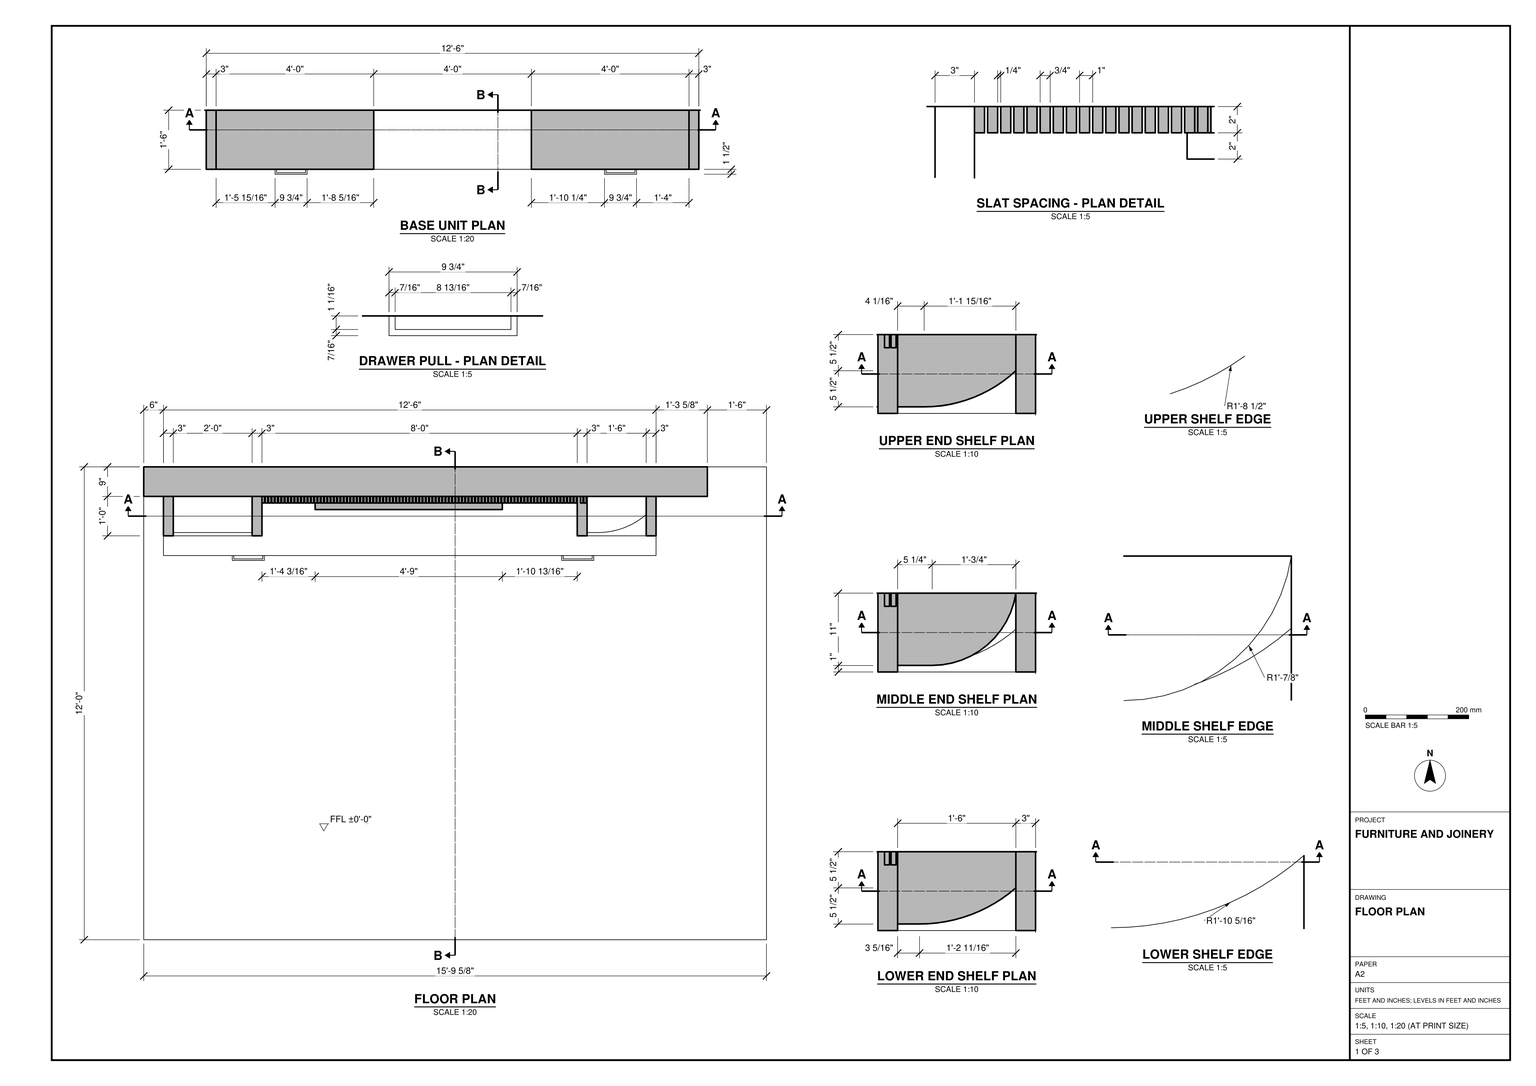
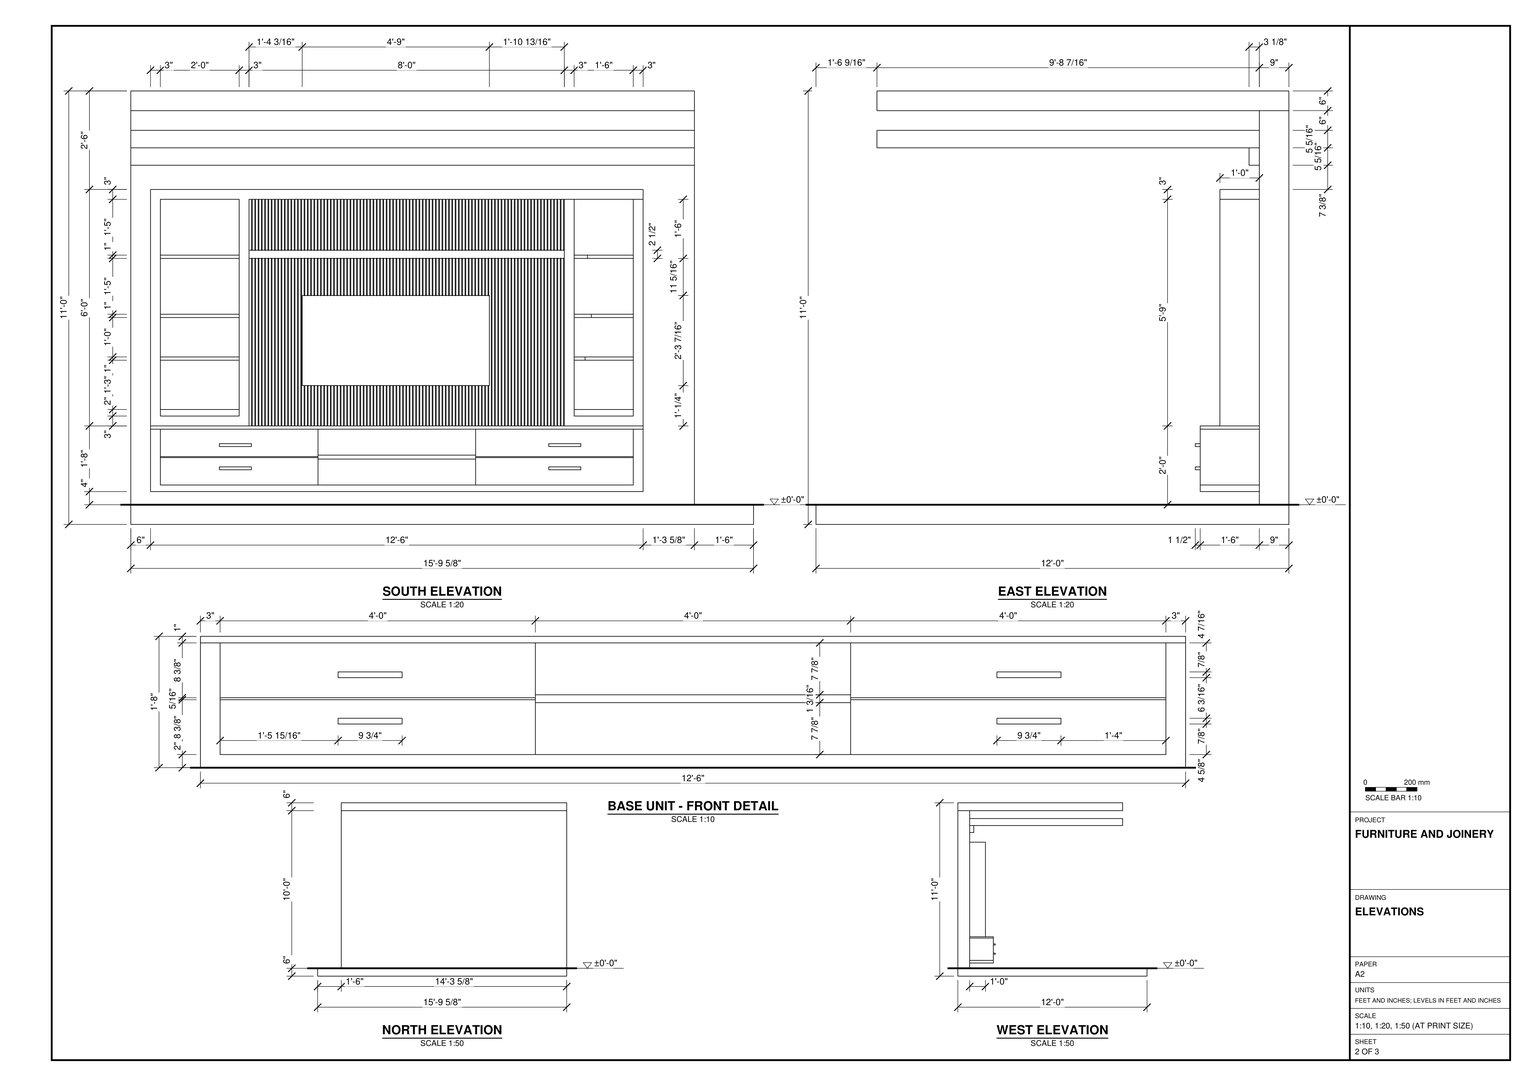
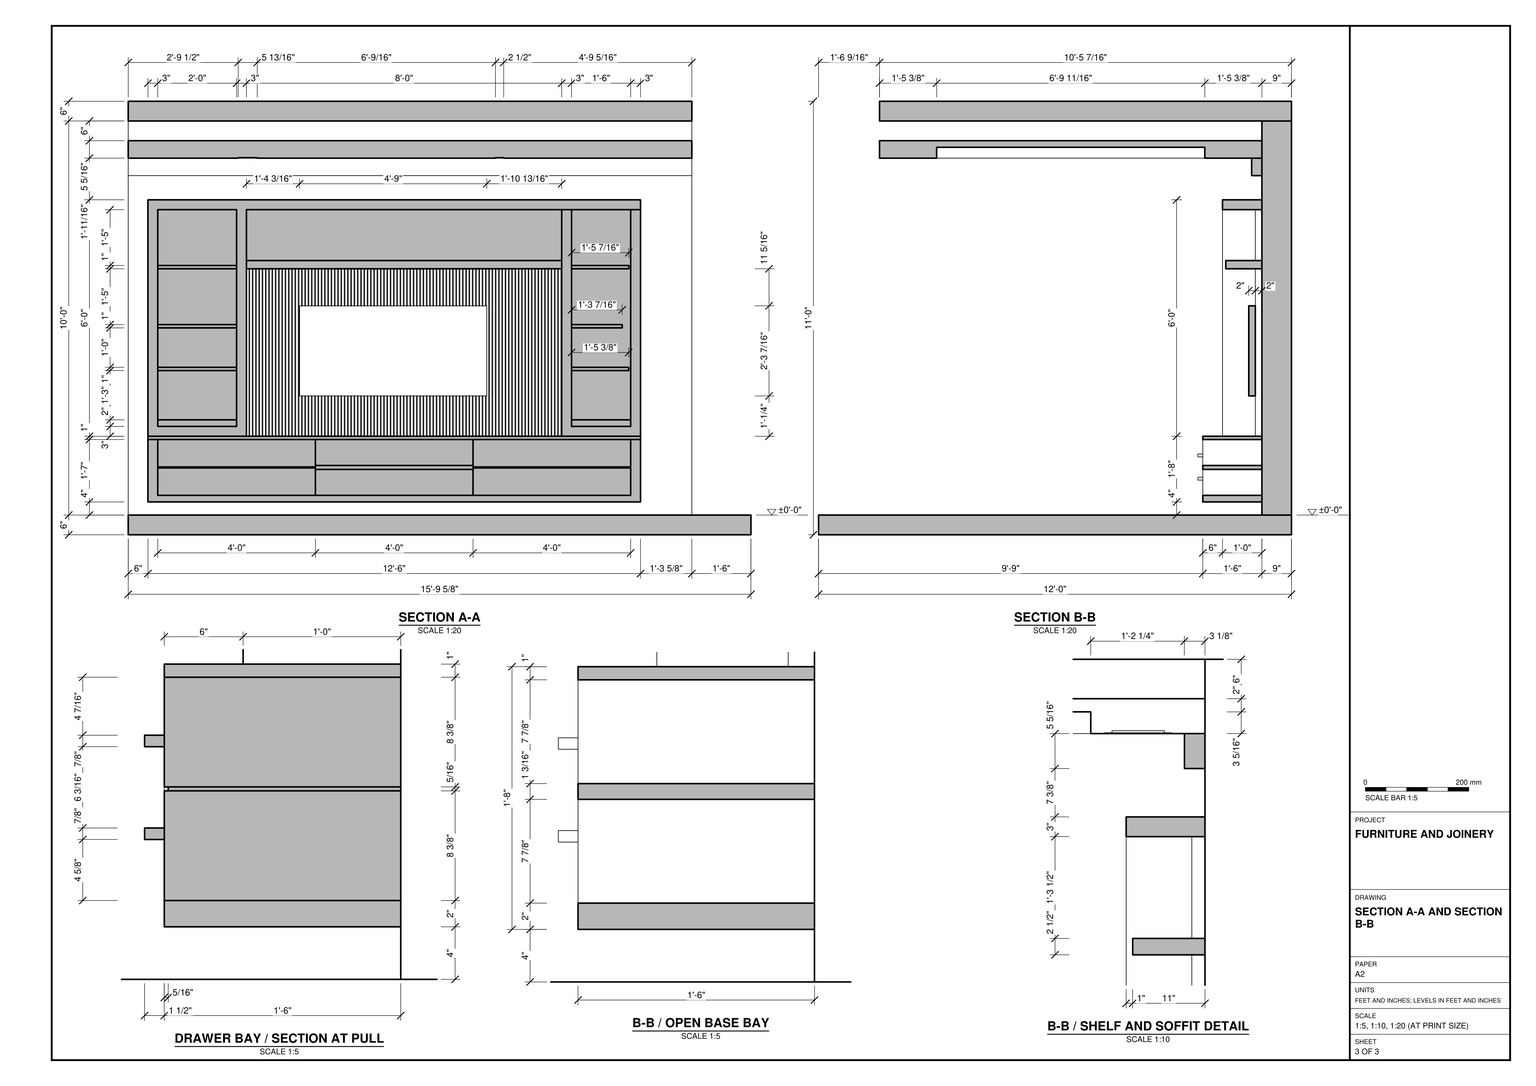
Build the TV wall unit and its architectural setting in SketchUp from task_files/diagram_01.pdf. Work in feet and inches. The complete model is 15'-9 5/8" wide, 12'-0" deep and 11'-0" high, with finished floor level at ±0'-0". Model the floor slab, the 9" backing wall, the overhead slab and the stepped soffit. Follow the floor plan for their offsets and section B-B for the soffit profile.

Set the base unit 4" above the finished floor. It is 12'-6" wide, with two stacked drawers in each outer bay and a shelf dividing the open middle bay. Model the projecting drawer pulls using the plan detail. Above the base, frame the vertical slat field between a wider shelving bay on the left and a narrower one on the right, as seen in the south elevation. Use the individual shelf plans for the curved edges on the right. Run a horizontal shelf across the slats above the TV screen, and position the screen as shown in the elevation.

Keep the shell elements and each furniture or joinery piece in separate groups or components, and use components for repeated parts. Decor and loose items may be any suitable library components. Save one SketchUp model as output_files/tv_wall_unit_with_slatted_backing_and_display_shelves.skp.

# SketchUp Ruby script. Lengths in inches.
U = 1.inch
M = Sketchup.active_model
def pt(a) = Geom::Point3d.new(a.map { |v| v * U })
def face(e, loops, mat)
  f = e.add_face(loops[0].map { |a| pt(a) })
  loops[1..].each { |l| e.add_face(l.map { |a| pt(a) }).erase! }
  f.material = f.back_material = mat if mat
  f
end
# faces: each face lists its corners as indices into pts; further lists are holes
def faces(e, pts, list, mat = nil) = list.each { |f| face(e, (f[0].is_a?(Array) ? f : [f]).map { |l| l.map { |i| pts[i] } }, mat) }
# xy, xz, yz: faces in a plane at the given z, y or x. An outline is a flat list of corners, or four numbers for a rectangle; further outlines are holes
def ring(l) = l.size == 4 ? [[l[0], l[1]], [l[2], l[1]], [l[2], l[3]], [l[0], l[3]]] : l.each_slice(2).to_a
def flat(e, list, mat, &to3) = list.each { |f| face(e, (f[0].is_a?(Array) ? f : [f]).map { |l| ring(l).map { |u, v| to3.(u, v) } }, mat) }
def xy(e, z, list, mat = nil) = flat(e, list, mat) { |x, y| [x, y, z] }
def xz(e, y, list, mat = nil) = flat(e, list, mat) { |x, z| [x, y, z] }
def yz(e, x, list, mat = nil) = flat(e, list, mat) { |y, z| [x, y, z] }
def lines(e, pts, list) = list.each { |a, b| e.add_line(pt(pts[a]), pt(pts[b])) }
# prism: a flat outline (further loops are holes) pulled along v
def prism(e, loops, v, mat = nil)
  f = face(e, loops, mat); d = Geom::Vector3d.new(v.map { |x| x * U })
  f.pushpull(f.normal.samedirection?(d) ? d.length : -d.length)
end
def box(e, o, s, mat = nil) = prism(e, [[o, [o[0] + s[0], o[1], o[2]], [o[0] + s[0], o[1] + s[1], o[2]], [o[0], o[1] + s[1], o[2]]]], [0, 0, s[2]], mat)
def at(x, y, z, deg = 0) = Geom::Transformation.translation(pt([x, y, z])) * Geom::Transformation.rotation(ORIGIN, Z_AXIS, deg.degrees)
def axes(o, x, y, z) = Geom::Transformation.new([*x, 0, *y, 0, *z, 0, *pt(o).to_a, 1])
def part(name) = M.definitions.add(name)
# library, detail: a bought-in or finely detailed component or shape, given as its bounding box
def library(name, o, s) = part(name).tap { |d| box(d.entities, o, s) }
def detail(e, o, s) = box(e.add_group.entities, o, s)
def put(e, d, t, mat = nil) = e.add_instance(d, t).tap { |i| i.material = mat if mat }
def group(e, t, mat = nil) = e.add_group.tap { |g| g.transformation = t; g.material = mat if mat }.entities
root = M.entities
M.materials.add("[Color D01]").color = [255, 242, 204]
M.materials.add("[Color E01]").color = [255, 255, 204]
M.materials.add("[Color M00]").color = [255, 255, 255]
M.materials.add("[Color M09]").color = [0, 0, 0]
M.materials.add("[Metal Aluminum Anodized]").color = [202, 209, 219]
M.materials.add("[Metal Silver]").color = [234, 233, 238]
M.materials.add("[Translucent Glass Gold]").color = [181, 87, 69]
M.materials["[Translucent Glass Gold]"].alpha = 0.6
M.materials.add("[Wood Cherry Original]").color = [152, 86, 42]
M.materials.add("[Wood Floor Light]").color = [204, 176, 127]
M.materials.add("[Wood Veneer 01]").color = [120, 70, 37]
c1 = part("Group\#16")
box(c1.entities,[0,0,0],[0.76,2,69])
c2 = part("Group\#21")
prism(c2.entities,[[[9.28,1.5,0],[9.75,1.5,0],[9.75,0,0],[0,0,0],[0,1.5,0],[0.47,1.5,0],[0.47,0.47,0],[9.28,0.47,0]]],[0,0,0.875])
g1 = group(root,at(0,0,0))
box(g1,[0,0,0],[189.625,144,6])
g2 = group(root,at(0,135,6),"[Color E01]")
box(g2,[0,0,0],[171.625,9,120])
g3 = group(root,at(6,123,30),"[Wood Veneer 01]")
prism(g3,[[[0,12,72],[150,12,72],[150,12,69],[30,12,69],[30,12,0],[0,12,0]],[[3,12,69],[3,12,3],[27,12,3],[27,12,69]]],[0,-12,0])
g4 = group(root,at(9,124,50),"[Translucent Glass Gold]")
box(g4,[0,0,0],[24,11,1])
g5 = group(root,at(9,124,63),"[Translucent Glass Gold]")
box(g5,[0,0,0],[24,11,1])
g6 = group(root,at(9,124,81),"[Translucent Glass Gold]")
box(g6,[0,0,0],[24,11,1])
g7 = group(root,at(9,123,33),"[Wood Floor Light]")
box(g7,[0,0,0],[24,12,2])
g8 = group(root,at(135,123,33),"[Wood Floor Light]")
box(g8,[0,0,0],[18,12,2])
g9 = group(root,at(36,124,81),"[Wood Veneer 01]")
box(g9,[0,0,0],[96,11,2.5])
g10 = group(root,at(6,117,29),"[Wood Cherry Original]")
box(g10,[0,0,0],[150,18,1])
g11 = group(root,at(6,117,10),"[Wood Cherry Original]")
xy(g11,0,[[0,0,150,18]])
xy(g11,2,[[3,0,147,18]])
xy(g11,19,[[0,0,3,18],[147,0,150,18]])
xz(g11,0,[[0,0,150,0,150,19,147,19,147,2,3,2,3,19,0,19]])
xz(g11,18,[[0,0,150,2],[0,2,3,19],[147,2,150,19]])
yz(g11,0,[[0,0,18,2],[0,2,18,19]])
yz(g11,3,[[0,2,18,19]])
yz(g11,147,[[0,2,18,19]])
yz(g11,150,[[0,0,18,2],[0,2,18,19]])
g12 = group(root,at(9,117,12),"[Wood Floor Light]")
xy(g12,0,[[0,0,48,18]])
xy(g12,8.35,[[0,0,48,0.3],[0,0.3,48,18]])
xy(g12,8.65,[[0,0,48,0.3],[0,0.3,48,18]])
xy(g12,17,[[0,0,48,18]])
xz(g12,0,[[0,0,48,8.35],[0,8.65,48,17]])
xz(g12,0.3,[[0,8.35,48,8.65]])
xz(g12,18,[[0,0,48,8.35],[0,8.35,48,8.65],[0,8.65,48,17]])
yz(g12,0,[[0,0,18,8.35],[0.3,8.35,18,8.65],[0,8.65,18,17]])
yz(g12,48,[[0,0,18,8.35],[0.3,8.35,18,8.65],[0,8.65,18,17]])
g13 = group(root,at(105,117,12),"[Wood Floor Light]")
xy(g13,0,[[0,0,48,18]])
xy(g13,8.35,[[0,0,48,0.3],[0,0.3,48,18]])
xy(g13,8.65,[[0,0,48,0.3],[0,0.3,48,18]])
xy(g13,17,[[0,0,48,18]])
xz(g13,0,[[0,0,48,8.35],[0,8.65,48,17]])
xz(g13,0.3,[[0,8.35,48,8.65]])
xz(g13,18,[[0,0,48,8.35],[0,8.35,48,8.65],[0,8.65,48,17]])
yz(g13,0,[[0,0,18,8.35],[0.3,8.35,18,8.65],[0,8.65,18,17]])
yz(g13,48,[[0,0,18,8.35],[0.3,8.35,18,8.65],[0,8.65,18,17]])
g14 = group(root,at(57,117,19.9),"[Wood Veneer 01]")
box(g14,[0,0,0],[48,18,1.2])
put(root,c1,at(36,133,30),"[Color D01]")
put(root,c1,at(37,133,30),"[Color D01]")
put(root,c1,at(38,133,30),"[Color D01]")
put(root,c1,at(39,133,30),"[Color D01]")
put(root,c1,at(40,133,30),"[Color D01]")
put(root,c1,at(41,133,30),"[Color D01]")
put(root,c1,at(42,133,30),"[Color D01]")
put(root,c1,at(43,133,30),"[Color D01]")
put(root,c1,at(44,133,30),"[Color D01]")
put(root,c1,at(45,133,30),"[Color D01]")
put(root,c1,at(46,133,30),"[Color D01]")
put(root,c1,at(47,133,30),"[Color D01]")
put(root,c1,at(48,133,30),"[Color D01]")
put(root,c1,at(49,133,30),"[Color D01]")
put(root,c1,at(50,133,30),"[Color D01]")
put(root,c1,at(51,133,30),"[Color D01]")
put(root,c1,at(52,133,30),"[Color D01]")
put(root,c1,at(53,133,30),"[Color D01]")
put(root,c1,at(54,133,30),"[Color D01]")
put(root,c1,at(55,133,30),"[Color D01]")
put(root,c1,at(56,133,30),"[Color D01]")
put(root,c1,at(57,133,30),"[Color D01]")
put(root,c1,at(58,133,30),"[Color D01]")
put(root,c1,at(59,133,30),"[Color D01]")
put(root,c1,at(60,133,30),"[Color D01]")
put(root,c1,at(61,133,30),"[Color D01]")
put(root,c1,at(62,133,30),"[Color D01]")
put(root,c1,at(63,133,30),"[Color D01]")
put(root,c1,at(64,133,30),"[Color D01]")
put(root,c1,at(65,133,30),"[Color D01]")
put(root,c1,at(66,133,30),"[Color D01]")
put(root,c1,at(67,133,30),"[Color D01]")
put(root,c1,at(68,133,30),"[Color D01]")
put(root,c1,at(69,133,30),"[Color D01]")
put(root,c1,at(70,133,30),"[Color D01]")
put(root,c1,at(71,133,30),"[Color D01]")
put(root,c1,at(72,133,30),"[Color D01]")
put(root,c1,at(73,133,30),"[Color D01]")
put(root,c1,at(74,133,30),"[Color D01]")
put(root,c1,at(75,133,30),"[Color D01]")
put(root,c1,at(76,133,30),"[Color D01]")
put(root,c1,at(77,133,30),"[Color D01]")
put(root,c1,at(78,133,30),"[Color D01]")
put(root,c1,at(79,133,30),"[Color D01]")
put(root,c1,at(80,133,30),"[Color D01]")
put(root,c1,at(81,133,30),"[Color D01]")
put(root,c1,at(82,133,30),"[Color D01]")
put(root,c1,at(83,133,30),"[Color D01]")
put(root,c1,at(84,133,30),"[Color D01]")
put(root,c1,at(85,133,30),"[Color D01]")
put(root,c1,at(86,133,30),"[Color D01]")
put(root,c1,at(87,133,30),"[Color D01]")
put(root,c1,at(88,133,30),"[Color D01]")
put(root,c1,at(89,133,30),"[Color D01]")
put(root,c1,at(90,133,30),"[Color D01]")
put(root,c1,at(91,133,30),"[Color D01]")
put(root,c1,at(92,133,30),"[Color D01]")
put(root,c1,at(93,133,30),"[Color D01]")
put(root,c1,at(94,133,30),"[Color D01]")
put(root,c1,at(95,133,30),"[Color D01]")
put(root,c1,at(96,133,30),"[Color D01]")
put(root,c1,at(97,133,30),"[Color D01]")
put(root,c1,at(98,133,30),"[Color D01]")
put(root,c1,at(99,133,30),"[Color D01]")
put(root,c1,at(100,133,30),"[Color D01]")
put(root,c1,at(101,133,30),"[Color D01]")
put(root,c1,at(102,133,30),"[Color D01]")
put(root,c1,at(103,133,30),"[Color D01]")
put(root,c1,at(104,133,30),"[Color D01]")
put(root,c1,at(105,133,30),"[Color D01]")
put(root,c1,at(106,133,30),"[Color D01]")
put(root,c1,at(107,133,30),"[Color D01]")
put(root,c1,at(108,133,30),"[Color D01]")
put(root,c1,at(109,133,30),"[Color D01]")
put(root,c1,at(110,133,30),"[Color D01]")
put(root,c1,at(111,133,30),"[Color D01]")
put(root,c1,at(112,133,30),"[Color D01]")
put(root,c1,at(113,133,30),"[Color D01]")
put(root,c1,at(114,133,30),"[Color D01]")
put(root,c1,at(115,133,30),"[Color D01]")
put(root,c1,at(116,133,30),"[Color D01]")
put(root,c1,at(117,133,30),"[Color D01]")
put(root,c1,at(118,133,30),"[Color D01]")
put(root,c1,at(119,133,30),"[Color D01]")
put(root,c1,at(120,133,30),"[Color D01]")
put(root,c1,at(121,133,30),"[Color D01]")
put(root,c1,at(122,133,30),"[Color D01]")
put(root,c1,at(123,133,30),"[Color D01]")
put(root,c1,at(124,133,30),"[Color D01]")
put(root,c1,at(125,133,30),"[Color D01]")
put(root,c1,at(126,133,30),"[Color D01]")
put(root,c1,at(127,133,30),"[Color D01]")
put(root,c1,at(128,133,30),"[Color D01]")
put(root,c1,at(129,133,30),"[Color D01]")
put(root,c1,at(130,133,30),"[Color D01]")
put(root,c1,at(131,133,30),"[Color D01]")
put(root,c1,at(133,133,30))
put(root,c1,at(134,133,30))
g15 = group(root,at(52.1875,131,42.27),"[Color M09]")
box(g15,[0,0,0],[57,2,27.44])
g16 = group(root,at(0,18.5625,118),"[Color E01]")
xy(g16,-3.3125,[[[0,0,171.625,116.4375],[17.39,17.39,154.24,99.05],[36.38,101.14,37.71,101.3125,38.94,101.82,40,102.64,40.82,103.7,41.33,104.94,41.5,106.26,41.33,107.59,40.82,108.82,40,109.89,38.94,110.7,37.71,111.21,36.38,111.39,35.05,111.21,33.82,110.7,32.75,109.89,31.94,108.82,31.43,107.59,31.25,106.26,31.43,104.94,31.94,103.7,32.75,102.64,33.82,101.82,35.05,101.3125],[113.08,100.98,114.32,101.15,115.48,101.63,116.48,102.39,117.25,103.39,117.73,104.55,117.89,105.8,117.73,107.04,117.25,108.2,116.48,109.2,115.48,109.96,114.32,110.44,113.08,110.61,111.83,110.44,110.67,109.96,109.67,109.2,108.91,108.2,108.43,107.04,108.27,105.8,108.43,104.55,108.91,103.39,109.67,102.39,110.67,101.63,111.83,101.15]]])
xy(g16,-3.1875,[[[113.08,100.98,111.83,101.15,110.67,101.63,109.67,102.39,108.91,103.39,108.43,104.55,108.27,105.8,108.43,107.04,108.91,108.2,109.67,109.2,110.67,109.96,111.83,110.44,113.08,110.61,114.32,110.44,115.48,109.96,116.48,109.2,117.25,108.2,117.73,107.04,117.89,105.8,117.73,104.55,117.25,103.39,116.48,102.39,115.48,101.63,114.32,101.15],[113.08,102.09,114.04,102.22,114.93,102.59,115.7,103.18,116.29,103.94,116.66,104.84,116.78,105.8,116.66,106.75,116.29,107.65,115.7,108.42,114.93,109,114.04,109.375,113.08,109.5,112.12,109.375,111.23,109,110.46,108.42,109.87,107.65,109.5,106.75,109.375,105.8,109.5,104.84,109.87,103.94,110.46,103.18,111.23,102.59,112.12,102.22]],[[36.38,101.14,35.05,101.3125,33.82,101.82,32.75,102.64,31.94,103.7,31.43,104.94,31.25,106.26,31.43,107.59,31.94,108.82,32.75,109.89,33.82,110.7,35.05,111.21,36.38,111.39,37.71,111.21,38.94,110.7,40,109.89,40.82,108.82,41.33,107.59,41.5,106.26,41.33,104.94,40.82,103.7,40,102.64,38.94,101.82,37.71,101.3125],[36.38,102.28,37.41,102.41,38.37,102.8125,39.2,103.44,39.83,104.27,40.23,105.23,40.36,106.26,40.23,107.29,39.83,108.25,39.2,109.08,38.37,109.71,37.41,110.11,36.38,110.25,35.35,110.11,34.39,109.71,33.5625,109.08,32.93,108.25,32.53,107.29,32.4,106.26,32.53,105.23,32.93,104.27,33.5625,103.44,34.39,102.8125,35.35,102.41]]],"[Metal Aluminum Anodized]")
xy(g16,-2.875,[[36.38,102.28,35.35,102.41,34.39,102.8125,33.5625,103.44,32.93,104.27,32.53,105.23,32.4,106.26,32.53,107.29,32.93,108.25,33.5625,109.08,34.39,109.71,35.35,110.11,36.38,110.25,37.41,110.11,38.37,109.71,39.2,109.08,39.83,108.25,40.23,107.29,40.36,106.26,40.23,105.23,39.83,104.27,39.2,103.44,38.37,102.8125,37.41,102.41]],"[Metal Silver]")
xy(g16,-2.8125,[[113.08,102.09,112.12,102.22,111.23,102.59,110.46,103.18,109.87,103.94,109.5,104.84,109.375,105.8,109.5,106.75,109.87,107.65,110.46,108.42,111.23,109,112.12,109.375,113.08,109.5,114.04,109.375,114.93,109,115.7,108.42,116.29,107.65,116.66,106.75,116.78,105.8,116.66,104.84,116.29,103.94,115.7,103.18,114.93,102.59,114.04,102.22]],"[Metal Silver]")
xy(g16,0,[[17.39,17.39,154.24,99.05]],"[Color M00]")
xy(g16,2,[[0,0,171.625,116.4375]])
xz(g16,0,[[0,-3.3125,171.625,2]])
xz(g16,17.39,[[17.39,-3.3125,154.24,0]])
xz(g16,99.05,[[17.39,-3.3125,154.24,0]])
xz(g16,116.4375,[[0,-3.3125,171.625,2]])
yz(g16,0,[[0,-3.3125,116.4375,2]])
yz(g16,17.39,[[17.39,-3.3125,99.05,0]])
yz(g16,154.24,[[17.39,-3.3125,99.05,0]])
yz(g16,171.625,[[0,-3.3125,116.4375,2]])
p = [[113.08,100.98,-3.3125],[111.83,101.15,-3.3125],[111.83,101.15,-3.1875],[113.08,100.98,-3.1875],[114.32,101.15,-3.3125],[114.32,101.15,-3.1875],
  [36.38,101.14,-3.3125],[35.05,101.3125,-3.3125],[35.05,101.3125,-3.1875],[36.38,101.14,-3.1875],[37.71,101.3125,-3.3125],[37.71,101.3125,-3.1875],
  [110.67,101.63,-3.3125],[110.67,101.63,-3.1875],[115.48,101.63,-3.3125],[115.48,101.63,-3.1875],[33.82,101.82,-3.3125],[33.82,101.82,-3.1875],
  [38.94,101.82,-3.3125],[38.94,101.82,-3.1875],[109.67,102.39,-3.3125],[109.67,102.39,-3.1875],[116.48,102.39,-3.3125],[116.48,102.39,-3.1875],
  [32.75,102.64,-3.3125],[32.75,102.64,-3.1875],[40,102.64,-3.3125],[40,102.64,-3.1875],[108.91,103.39,-3.3125],[108.91,103.39,-3.1875],
  [117.25,103.39,-3.3125],[117.25,103.39,-3.1875],[31.94,103.7,-3.3125],[31.94,103.7,-3.1875],[40.82,103.7,-3.3125],[40.82,103.7,-3.1875],
  [108.43,104.55,-3.3125],[108.43,104.55,-3.1875],[117.73,104.55,-3.3125],[117.73,104.55,-3.1875],[31.43,104.94,-3.3125],[31.43,104.94,-3.1875],
  [41.33,104.94,-3.3125],[41.33,104.94,-3.1875],[108.27,105.8,-3.3125],[108.27,105.8,-3.1875],[117.89,105.8,-3.3125],[117.89,105.8,-3.1875],
  [31.25,106.26,-3.3125],[31.25,106.26,-3.1875],[41.5,106.26,-3.3125],[41.5,106.26,-3.1875],[108.43,107.04,-3.3125],[108.43,107.04,-3.1875],
  [117.73,107.04,-3.3125],[117.73,107.04,-3.1875],[31.43,107.59,-3.3125],[31.43,107.59,-3.1875],[41.33,107.59,-3.3125],[41.33,107.59,-3.1875],
  [108.91,108.2,-3.3125],[108.91,108.2,-3.1875],[117.25,108.2,-3.3125],[117.25,108.2,-3.1875],[31.94,108.82,-3.3125],[31.94,108.82,-3.1875],
  [40.82,108.82,-3.3125],[40.82,108.82,-3.1875],[109.67,109.2,-3.3125],[109.67,109.2,-3.1875],[116.48,109.2,-3.3125],[116.48,109.2,-3.1875],
  [32.75,109.89,-3.3125],[32.75,109.89,-3.1875],[40,109.89,-3.3125],[40,109.89,-3.1875],[110.67,109.96,-3.3125],[110.67,109.96,-3.1875],
  [115.48,109.96,-3.3125],[115.48,109.96,-3.1875],[33.82,110.7,-3.3125],[33.82,110.7,-3.1875],[38.94,110.7,-3.3125],[38.94,110.7,-3.1875],
  [111.83,110.44,-3.3125],[111.83,110.44,-3.1875],[114.32,110.44,-3.3125],[114.32,110.44,-3.1875],[113.08,110.61,-3.3125],[113.08,110.61,-3.1875],
  [35.05,111.21,-3.3125],[35.05,111.21,-3.1875],[37.71,111.21,-3.3125],[37.71,111.21,-3.1875],[36.38,111.39,-3.3125],[36.38,111.39,-3.1875],
  [113.08,102.09,-2.8125],[113.08,102.09,-3.1875],[112.12,102.22,-3.1875],[112.12,102.22,-2.8125],[114.04,102.22,-2.8125],[114.04,102.22,-3.1875],
  [111.23,102.59,-3.1875],[111.23,102.59,-2.8125],[114.93,102.59,-2.8125],[114.93,102.59,-3.1875],[36.38,102.28,-2.875],[36.38,102.28,-3.1875],
  [35.35,102.41,-3.1875],[35.35,102.41,-2.875],[37.41,102.41,-2.875],[37.41,102.41,-3.1875],[34.39,102.8125,-3.1875],[34.39,102.8125,-2.875],
  [38.37,102.8125,-2.875],[38.37,102.8125,-3.1875],[110.46,103.18,-3.1875],[110.46,103.18,-2.8125],[115.7,103.18,-2.8125],[115.7,103.18,-3.1875],
  [33.5625,103.44,-3.1875],[33.5625,103.44,-2.875],[39.2,103.44,-2.875],[39.2,103.44,-3.1875],[109.87,103.94,-3.1875],[109.87,103.94,-2.8125],
  [116.29,103.94,-2.8125],[116.29,103.94,-3.1875],[32.93,104.27,-3.1875],[32.93,104.27,-2.875],[39.83,104.27,-2.875],[39.83,104.27,-3.1875],
  [109.5,104.84,-3.1875],[109.5,104.84,-2.8125],[116.66,104.84,-2.8125],[116.66,104.84,-3.1875],[32.53,105.23,-3.1875],[32.53,105.23,-2.875],
  [40.23,105.23,-2.875],[40.23,105.23,-3.1875],[109.375,105.8,-3.1875],[109.375,105.8,-2.8125],[116.78,105.8,-2.8125],[116.78,105.8,-3.1875],
  [32.4,106.26,-3.1875],[32.4,106.26,-2.875],[40.36,106.26,-2.875],[40.36,106.26,-3.1875],[109.5,106.75,-3.1875],[109.5,106.75,-2.8125],
  [116.66,106.75,-2.8125],[116.66,106.75,-3.1875],[32.53,107.29,-3.1875],[32.53,107.29,-2.875],[40.23,107.29,-2.875],[40.23,107.29,-3.1875],
  [109.87,107.65,-3.1875],[109.87,107.65,-2.8125],[116.29,107.65,-2.8125],[116.29,107.65,-3.1875],[32.93,108.25,-3.1875],[32.93,108.25,-2.875],
  [39.83,108.25,-2.875],[39.83,108.25,-3.1875],[110.46,108.42,-3.1875],[110.46,108.42,-2.8125],[115.7,108.42,-2.8125],[115.7,108.42,-3.1875],
  [33.5625,109.08,-3.1875],[33.5625,109.08,-2.875],[39.2,109.08,-2.875],[39.2,109.08,-3.1875],[111.23,109,-3.1875],[111.23,109,-2.8125],
  [114.93,109,-2.8125],[114.93,109,-3.1875],[112.12,109.375,-3.1875],[112.12,109.375,-2.8125],[114.04,109.375,-2.8125],[114.04,109.375,-3.1875],
  [34.39,109.71,-3.1875],[34.39,109.71,-2.875],[38.37,109.71,-2.875],[38.37,109.71,-3.1875],[113.08,109.5,-3.1875],[113.08,109.5,-2.8125],
  [35.35,110.11,-3.1875],[35.35,110.11,-2.875],[37.41,110.11,-2.875],[37.41,110.11,-3.1875],[36.38,110.25,-3.1875],[36.38,110.25,-2.875]]
faces(g16,p,[[0,1,2,3],[4,0,3,5],[6,7,8,9],[10,6,9,11],[1,12,13,2],[14,4,5,15],[7,16,17,8],[18,10,11,19],
  [12,20,21,13],[22,14,15,23],[16,24,25,17],[26,18,19,27],[20,28,29,21],[30,22,23,31],[24,32,33,25],[34,26,27,35],
  [28,36,37,29],[38,30,31,39],[32,40,41,33],[42,34,35,43],[36,44,45,37],[46,38,39,47],[40,48,49,41],[50,42,43,51],
  [44,52,53,45],[54,46,47,55],[48,56,57,49],[58,50,51,59],[52,60,61,53],[62,54,55,63],[56,64,65,57],[66,58,59,67],
  [60,68,69,61],[70,62,63,71],[64,72,73,65],[74,66,67,75],[68,76,77,69],[78,70,71,79],[72,80,81,73],[82,74,75,83],
  [76,84,85,77],[86,78,79,87],[84,88,89,85],[88,86,87,89],[80,90,91,81],[92,82,83,93],[90,94,95,91],[94,92,93,95]])
faces(g16,p,[[96,97,98,99],[100,101,97,96],[99,98,102,103],[104,105,101,100],[106,107,108,109],[110,111,107,106],[109,108,112,113],[114,115,111,110],
  [103,102,116,117],[118,119,105,104],[113,112,120,121],[122,123,115,114],[117,116,124,125],[126,127,119,118],[121,120,128,129],[130,131,123,122],
  [125,124,132,133],[134,135,127,126],[129,128,136,137],[138,139,131,130],[133,132,140,141],[142,143,135,134],[137,136,144,145],[146,147,139,138],
  [141,140,148,149],[150,151,143,142],[145,144,152,153],[154,155,147,146],[149,148,156,157],[158,159,151,150],[153,152,160,161],[162,163,155,154],
  [157,156,164,165],[166,167,159,158],[161,160,168,169],[170,171,163,162],[165,164,172,173],[174,175,167,166],[173,172,176,177],[178,179,175,174],
  [169,168,180,181],[182,183,171,170],[177,176,184,185],[185,184,179,178],[181,180,186,187],[188,189,183,182],[187,186,190,191],[191,190,189,188]],"[Metal Aluminum Anodized]")
g17 = group(root,at(0,131.875,109.37),"[Wood Veneer 01]")
box(g17,[0,0,0],[171.625,3.125,5.32])
g18 = group(root,at(0,18.5625,126))
box(g18,[0,0,0],[171.625,125.4375,6])
put(root,c2,at(26.96,115.5,16.65),"[Metal Aluminum Anodized]")
put(root,c2,at(26.96,115.5,23.71),"[Metal Aluminum Anodized]")
put(root,c2,at(127.28,115.5,23.71),"[Metal Aluminum Anodized]")
put(root,c2,at(127.28,115.5,16.65),"[Metal Aluminum Anodized]")
g19 = group(root,at(132,123,30))
xy(g19,0,[[0,0,3,12],[3,0,21,12],[21,0,24,12]],"[Wood Veneer 01]")
xy(g19,3,[[3,0,21,12]],"[Wood Veneer 01]")
xy(g19,20,[[3,1,3,12,21,12,21,6.5,19.97,5.65,18.89,4.87,17.76,4.15,16.6,3.5,15.39,2.93,14.16,2.42,12.9,1.99,11.61,1.63,10.3,1.36,8.98,1.16,7.66,1.04,6.32,1]],"[Translucent Glass Gold]")
xy(g19,21,[[3,1,6.32,1,7.66,1.04,8.98,1.16,10.3,1.36,11.61,1.63,12.9,1.99,14.16,2.42,15.39,2.93,16.6,3.5,17.76,4.15,18.89,4.87,19.97,5.65,21,6.5,21,12,3,12]],"[Translucent Glass Gold]")
xy(g19,33,[[3,1,3,12,21,12,20.6875,10.5,20.2,9.06,19.54,7.68,18.72,6.38,17.76,5.19,16.67,4.13,15.45,3.2,14.13,2.42,12.74,1.81,11.27,1.36,9.77,1.09,8.24,1]],"[Translucent Glass Gold]")
xy(g19,34,[[3,1,8.24,1,9.77,1.09,11.27,1.36,12.74,1.81,14.13,2.42,15.45,3.2,16.67,4.13,17.76,5.19,18.72,6.38,19.54,7.68,20.2,9.06,20.6875,10.5,21,12,3,12]],"[Translucent Glass Gold]")
xy(g19,51,[[3,1,3,12,21,12,21,6.5,20.04,5.66,19.02,4.875,17.96,4.16,16.85,3.51,15.71,2.93,14.53,2.42,13.33,1.99,12.1,1.64,10.85,1.36,9.58,1.16,8.31,1.04,7.03,1]],"[Translucent Glass Gold]")
xy(g19,52,[[3,1,7.03,1,8.31,1.04,9.58,1.16,10.85,1.36,12.1,1.64,13.33,1.99,14.53,2.42,15.71,2.93,16.85,3.51,17.96,4.16,19.02,4.875,20.04,5.66,21,6.5,21,12,3,12]],"[Translucent Glass Gold]")
xy(g19,69,[[0,0,3,12],[21,0,24,12]],"[Wood Veneer 01]")
xz(g19,0,[[0,0,24,0,24,69,21,69,21,3,3,3,3,69,0,69]],"[Wood Veneer 01]")
xz(g19,1,[[3,20,6.32,21],[3,33,8.24,34],[3,51,7.03,52]],"[Translucent Glass Gold]")
xz(g19,12,[[0,0,3,69],[3,0,21,3],[21,0,24,69],[3,20,21,21],[3,33,21,34],
  [3,51,21,52]],"[Wood Veneer 01]")
yz(g19,0,[[0,0,12,69]],"[Wood Veneer 01]")
yz(g19,3,[[0,3,12,3,12,20,1,20,1,21,12,21,12,33,1,33,1,34,12,34,12,51,1,51,1,52,12,52,12,69,0,69],[1,20,12,21],[1,33,12,34],[1,51,12,52]],"[Wood Veneer 01]")
yz(g19,21,[[0,3,0,69,12,69,12,52,6.5,52,6.5,51,12,51,12,21,6.5,21,6.5,20,12,20,12,3],[6.5,20,12,21],[6.5,51,12,52]],"[Wood Veneer 01]")
yz(g19,24,[[0,0,12,69]],"[Wood Veneer 01]")
p = [[7.66,1.04,21],[6.32,1,21],[6.32,1,20],[7.66,1.04,20],[8.98,1.16,21],[8.98,1.16,20],
  [10.3,1.36,21],[10.3,1.36,20],[11.61,1.63,21],[11.61,1.63,20],[12.9,1.99,21],[12.9,1.99,20],
  [14.16,2.42,21],[14.16,2.42,20],[15.39,2.93,21],[15.39,2.93,20],[16.6,3.5,21],[16.6,3.5,20],
  [17.76,4.15,21],[17.76,4.15,20],[18.89,4.87,21],[18.89,4.87,20],[19.97,5.65,21],[19.97,5.65,20],
  [21,6.5,21],[21,6.5,20],[9.77,1.09,34],[8.24,1,34],[8.24,1,33],[9.77,1.09,33],
  [11.27,1.36,34],[11.27,1.36,33],[12.74,1.81,34],[12.74,1.81,33],[14.13,2.42,34],[14.13,2.42,33],
  [15.45,3.2,34],[15.45,3.2,33],[16.67,4.13,34],[16.67,4.13,33],[17.76,5.19,34],[17.76,5.19,33],
  [18.72,6.38,34],[18.72,6.38,33],[19.54,7.68,34],[19.54,7.68,33],[20.2,9.06,34],[20.2,9.06,33],
  [20.6875,10.5,34],[20.6875,10.5,33],[21,12,34],[21,12,33],[8.31,1.04,52],[7.03,1,52],
  [7.03,1,51],[8.31,1.04,51],[9.58,1.16,52],[9.58,1.16,51],[10.85,1.36,52],[10.85,1.36,51],
  [12.1,1.64,52],[12.1,1.64,51],[13.33,1.99,52],[13.33,1.99,51],[14.53,2.42,52],[14.53,2.42,51],
  [15.71,2.93,52],[15.71,2.93,51],[16.85,3.51,52],[16.85,3.51,51],[17.96,4.16,52],[17.96,4.16,51],
  [19.02,4.875,52],[19.02,4.875,51],[20.04,5.66,52],[20.04,5.66,51],[21,6.5,52],[21,6.5,51]]
faces(g19,p,[[0,1,2,3],[4,0,3,5],[6,4,5,7],[8,6,7,9],[10,8,9,11],[12,10,11,13],[14,12,13,15],[16,14,15,17],
  [18,16,17,19],[20,18,19,21],[22,20,21,23],[24,22,23,25],[26,27,28,29],[30,26,29,31],[32,30,31,33],[34,32,33,35],
  [36,34,35,37],[38,36,37,39],[40,38,39,41],[42,40,41,43],[44,42,43,45],[46,44,45,47],[48,46,47,49],[50,48,49,51],
  [52,53,54,55],[56,52,55,57],[58,56,57,59],[60,58,59,61],[62,60,61,63],[64,62,63,65],[66,64,65,67],[68,66,67,69],
  [70,68,69,71],[72,70,71,73],[74,72,73,75],[76,74,75,77]],"[Translucent Glass Gold]")
